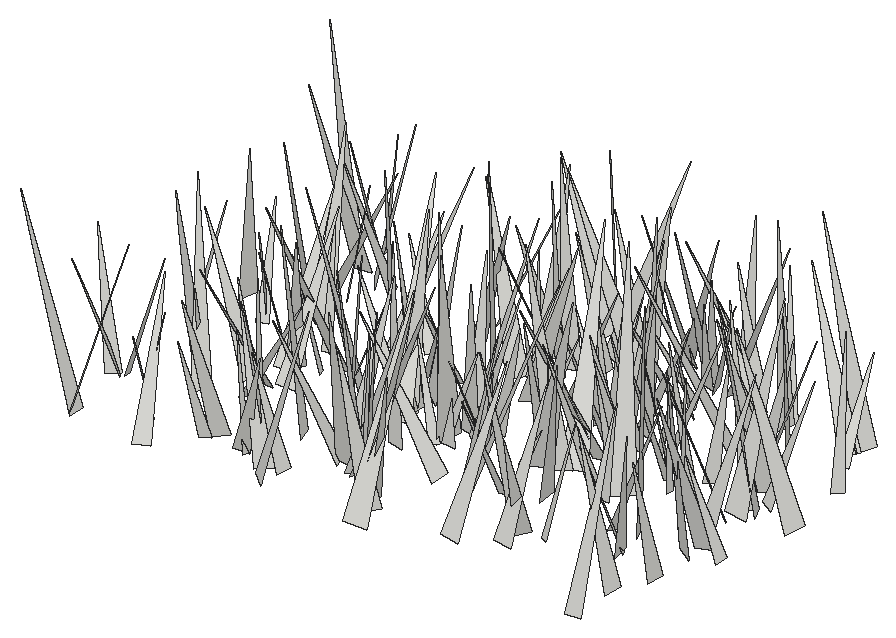
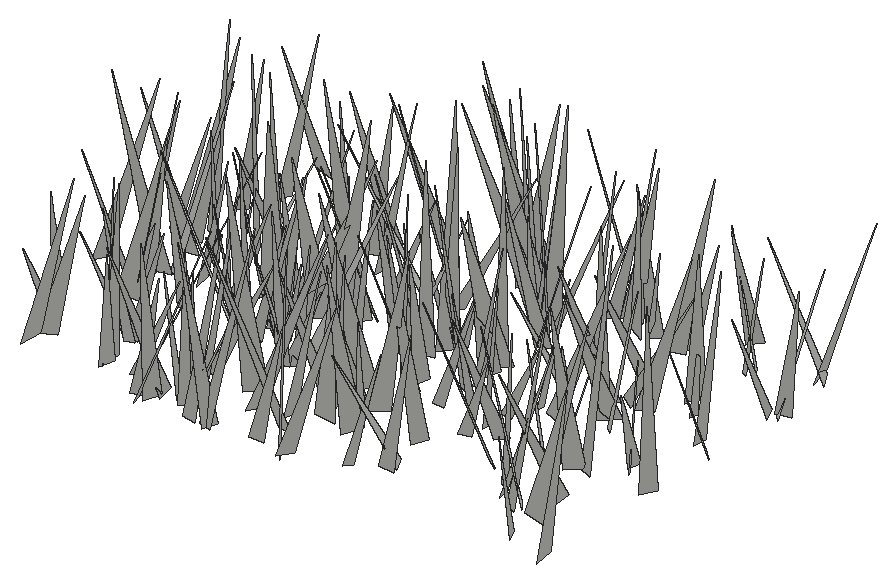
# SketchUp Ruby script. Lengths in inches.
U = 1.inch
M = Sketchup.active_model
def pt(a) = Geom::Point3d.new(a.map { |v| v * U })
def face(e, loops, mat)
  f = e.add_face(loops[0].map { |a| pt(a) })
  loops[1..].each { |l| e.add_face(l.map { |a| pt(a) }).erase! }
  f.material = f.back_material = mat if mat
  f
end
# faces: each face lists its corners as indices into pts; further lists are holes
def faces(e, pts, list, mat = nil) = list.each { |f| face(e, (f[0].is_a?(Array) ? f : [f]).map { |l| l.map { |i| pts[i] } }, mat) }
# xy, xz, yz: faces in a plane at the given z, y or x. An outline is a flat list of corners, or four numbers for a rectangle; further outlines are holes
def ring(l) = l.size == 4 ? [[l[0], l[1]], [l[2], l[1]], [l[2], l[3]], [l[0], l[3]]] : l.each_slice(2).to_a
def flat(e, list, mat, &to3) = list.each { |f| face(e, (f[0].is_a?(Array) ? f : [f]).map { |l| ring(l).map { |u, v| to3.(u, v) } }, mat) }
def xy(e, z, list, mat = nil) = flat(e, list, mat) { |x, y| [x, y, z] }
def xz(e, y, list, mat = nil) = flat(e, list, mat) { |x, z| [x, y, z] }
def yz(e, x, list, mat = nil) = flat(e, list, mat) { |y, z| [x, y, z] }
def lines(e, pts, list) = list.each { |a, b| e.add_line(pt(pts[a]), pt(pts[b])) }
# prism: a flat outline (further loops are holes) pulled along v
def prism(e, loops, v, mat = nil)
  f = face(e, loops, mat); d = Geom::Vector3d.new(v.map { |x| x * U })
  f.pushpull(f.normal.samedirection?(d) ? d.length : -d.length)
end
def box(e, o, s, mat = nil) = prism(e, [[o, [o[0] + s[0], o[1], o[2]], [o[0] + s[0], o[1] + s[1], o[2]], [o[0], o[1] + s[1], o[2]]]], [0, 0, s[2]], mat)
def at(x, y, z, deg = 0) = Geom::Transformation.translation(pt([x, y, z])) * Geom::Transformation.rotation(ORIGIN, Z_AXIS, deg.degrees)
def axes(o, x, y, z) = Geom::Transformation.new([*x, 0, *y, 0, *z, 0, *pt(o).to_a, 1])
def part(name) = M.definitions.add(name)
# library, detail: a bought-in or finely detailed component or shape, given as its bounding box
def library(name, o, s) = part(name).tap { |d| box(d.entities, o, s) }
def detail(e, o, s) = box(e.add_group.entities, o, s)
def put(e, d, t, mat = nil) = e.add_instance(d, t).tap { |i| i.material = mat if mat }
def group(e, t, mat = nil) = e.add_group.tap { |g| g.transformation = t; g.material = mat if mat }.entities
root = M.entities
c1 = part("fur_instance\#9")
p = [[0.8125,0,1.79],[0.67,-0.02,1.48],[0,-0.11,0],[0,0.11,0]]
faces(c1.entities,p,[[0,1,2,3]])
put(root,c1,axes([455.83,105.99,-21.66],[-7.51977,-1.08655,0.44758],[-1.14316,7.43533,-1.15625],[0.27218,1.20961,7.50937]))
put(root,c1,axes([478.6,107.64,-21.66],[3.4747,-4.84053,2.29693],[-4.84614,-4.00697,-1.11322],[-2.28507,1.13736,5.85363]))
put(root,c1,axes([470.41,106.39,-21.66],[4.17066,5.06918,1.33611],[5.23853,-4.09478,-0.81653],[-0.19883,-1.55319,6.51339]))
put(root,c1,axes([461.78,105.19,-21.66],[-3.2921,4.67046,0.35788],[4.62081,3.30978,-0.68745],[0.76768,0.10645,5.67261]))
put(root,c1,axes([478.07,108.55,-21.66],[6.05752,-0.57817,0.88939],[-0.39,-6.0087,-1.2499],[-0.9865,-1.17476,5.9553]))
put(root,c1,axes([459.88,108.68,-21.66],[-2.01295,-3.23513,0.63988],[-3.06607,2.112,1.03257],[1.21439,-0.03018,3.66768]))
put(root,c1,axes([467.22,108.6,-21.66],[2.01974,-4.62687,0.27657],[-4.52399,-1.90214,1.21619],[1.00891,0.73329,4.89981]))
put(root,c1,axes([459.48,107.97,-21.66],[4.05743,2.55482,1.17911],[2.80714,-3.81746,-1.3882],[-0.19333,-1.81108,4.58942]))
put(root,c1,axes([471.05,108.2,-21.66],[3.41803,-2.18502,2.15563],[-1.95303,-4.03718,-0.99543],[-2.36786,0.1758,3.93273]))
put(root,c1,axes([465.02,109.28,-21.66],[2.93992,-5.13493,1.13143],[-5.01799,-3.12719,-1.15379],[-1.5708,0.37938,5.8034]))
put(root,c1,axes([464.36,108.5,-21.66],[0.87067,-3.63818,0.96208],[-3.64876,-1.05785,-0.69825],[-0.92116,0.75142,3.67517]))
put(root,c1,axes([455.3125,106.12,-21.66],[5.06961,3.19969,0.78256],[3.08145,-5.11429,0.94868],[-1.16407,0.39664,5.91937]))
put(root,c1,axes([497.24,104.99,-21.66],[1.20703,6.81999,0.05967],[6.70849,-1.19813,1.23829],[-1.22962,0.158,6.81439]))
put(root,c1,axes([469.2,109.23,-21.66],[-5.69321,-2.11736,2.09192],[-1.78965,6.04293,1.24584],[2.37833,-0.52131,5.94506]))
put(root,c1,axes([478.99,105.47,-21.66],[-1.14842,8.02715,0.79991],[8.02073,1.22255,-0.75306],[0.86188,-0.68125,8.07384]))
put(root,c1,axes([478,107.31,-21.66],[7.83085,1.1219,1.78667],[1.00117,-8.02181,0.64907],[-1.85702,0.40616,7.88414]))
put(root,c1,axes([478.03,107.39,-21.66],[2.88835,4.68484,1.93004],[4.79823,-3.24275,0.69058],[-1.62782,-1.24585,5.46016]))
put(root,c1,axes([469.86,107.73,-21.66],[-2.9661,5.6248,1.68099],[5.86235,2.73802,1.18234],[-0.31135,-2.03143,6.24805]))
put(root,c1,axes([497.25,109.08,-21.66],[-5.83631,0.9789,1.84731],[1.28037,6.00401,0.86359],[1.65271,-1.19453,5.85448]))
put(root,c1,axes([476.66,109.51,-21.66],[6.37942,2.61315,2.43113],[3.05762,-6.56979,-0.96169],[-1.84118,-1.85616,6.82648]))
put(root,c1,axes([473.53,111.4,-21.66],[0.50064,-7.21064,0.91051],[-7.21991,-0.3887,0.89157],[0.83387,0.96363,7.17281]))
put(root,c1,axes([467.76,108.44,-21.66],[-4.02809,-0.22088,0.67447],[-0.39433,3.92835,-1.06856],[0.59008,1.11738,3.89005]))
put(root,c1,axes([488.08,111.35,-21.66],[3.42227,-3.49613,0.30492],[-3.40506,-3.41104,-0.89344],[-0.84941,-0.41195,4.81005]))
put(root,c1,axes([484.82,107.88,-21.66],[0.10942,6.44965,1.02032],[6.44115,0.06102,-1.07648],[1.07264,-1.02435,6.36012]))
put(root,c1,axes([468.54,108.96,-21.66],[2.01081,5.29668,2.07869],[5.40677,-2.46554,1.0522],[-1.77275,-1.51176,5.56697]))
put(root,c1,axes([454.66,111.86,-21.66],[-3.71629,-3.62879,0.54604],[-3.4741,3.72939,1.13989],[1.18191,-0.44788,5.0675]))
put(root,c1,axes([472.95,111.67,-21.66],[-5.60277,-1.40853,0.55452],[-1.25772,5.51462,1.29985],[0.84237,-1.13469,5.62898]))
put(root,c1,axes([474.89,110.81,-21.66],[5.41416,-4.66063,0.97473],[-4.76032,-5.26587,1.26282],[0.1044,1.59183,7.03135]))
put(root,c1,axes([487.88,109.47,-21.66],[-0.68675,5.73435,1.62653],[5.78722,1.03346,-1.2],[1.42703,-1.4315,5.64928]))
put(root,c1,axes([498.39,111.98,-21.66],[4.51587,-1.82573,1.61231],[-1.49442,-4.75873,-1.20297],[-1.92343,-0.58918,4.72009]))
put(root,c1,axes([484.13,109.28,-21.66],[4.06792,5.19434,1.22411],[5.14399,-4.22635,0.83955],[-1.42088,-0.42943,6.54403]))
put(root,c1,axes([454.54,111.4,-21.66],[-2.06507,4.56305,1.47225],[4.79287,1.92061,0.77009],[-0.13147,-1.65628,4.94903]))
put(root,c1,axes([474.97,110.89,-21.66],[7.79072,-0.23447,0.87822],[-0.35324,-7.76347,1.06082],[-0.83754,1.09323,7.72172]))
put(root,c1,axes([486.36,112.78,-21.66],[-6.02473,-0.71032,1.74625],[-0.51818,6.24626,0.75302],[1.81257,-0.57532,6.01954]))
put(root,c1,axes([494.53,113.22,-21.66],[5.27182,0.13194,1.25121],[0.40362,-5.28245,-1.14356],[-1.19165,-1.2055,5.14798]))
put(root,c1,axes([474.9,111.47,-21.66],[-4.32916,0.66549,1.27706],[0.40908,4.44763,-0.93094],[1.38073,0.76884,4.27993]))
put(root,c1,axes([474.12,112.22,-21.66],[-5.98871,-2.33617,1.80164],[-2.60473,6.10133,-0.74665],[1.38529,1.37273,6.38474]))
put(root,c1,axes([472.31,113.12,-21.66],[5.33637,4.77614,2.80857],[5.34994,-5.45601,-0.88678],[-1.44141,-2.56842,7.10647]))
put(root,c1,axes([469.09,112.7,-21.66],[-6.68963,-2.36331,2.10659],[-2.62997,6.88987,-0.62215],[1.76244,1.31094,7.06748]))
put(root,c1,axes([479.42,113.69,-21.66],[-6.11827,1.22354,0.04324],[1.20265,5.96505,1.37981],[-0.22923,-1.36132,6.08493]))
put(root,c1,axes([455.33,111.8,-21.66],[3.79033,1.52401,0.8214],[1.29616,-3.80865,1.0854],[-1.14773,0.73179,3.93842]))
put(root,c1,axes([489.63,111.56,-21.66],[2.15657,3.40289,0.33157],[3.29952,-2.17412,0.8525],[-0.89598,0.18416,3.93747]))
put(root,c1,axes([494.66,113.41,-21.66],[-3.19994,-2.12817,0.10035],[-2.08753,3.09569,-0.91527],[-0.42587,0.81635,3.73243]))
put(root,c1,axes([483.8,114.61,-21.66],[-1.02707,-3.52995,0.46815],[-3.49734,0.90838,-0.82343],[-0.66956,0.66999,3.58293]))
put(root,c1,axes([458.94,115,-21.66],[3.4639,-0.21189,1.20284],[0.06017,-3.58323,-0.80448],[-1.21988,-0.7784,3.37584]))
put(root,c1,axes([497.77,115.72,-21.66],[-3.27673,-6.38483,2.25273],[-6.55108,3.62196,0.73666],[1.71005,1.64109,7.13865]))
put(root,c1,axes([462.99,114.27,-21.66],[4.12414,-1.44643,0.07491],[-1.4095,-3.95608,1.21201],[0.33327,1.1677,4.19901]))
put(root,c1,axes([486.26,116.03,-21.66],[6.1777,-0.38175,1.16241],[-0.13775,-6.16226,-1.29169],[-1.21571,-1.24165,6.0532]))
put(root,c1,axes([498.44,117.05,-21.66],[1.25653,-6.81976,0.6894],[-6.81087,-1.32116,-0.65555],[-0.77223,0.55558,6.90349]))
put(root,c1,axes([460.31,113.14,-21.66],[-6.55915,2.85076,0.80174],[2.70921,6.56329,-1.17278],[1.19574,0.76707,7.05506]))
put(root,c1,axes([472.05,114.02,-21.66],[-0.35457,5.93898,1.63328],[6.05839,0.63143,-0.98081],[1.11129,-1.54746,5.86815]))
put(root,c1,axes([463.4,116.24,-21.66],[-2.21504,-4.22644,0.02495],[-4.06696,2.12371,-1.31133],[-1.15036,0.62998,4.58799]))
put(root,c1,axes([500.15,116.52,-21.66],[-3.89042,0.9571,1.21715],[1.27935,3.84105,1.06884],[0.87221,-1.36496,3.86121]))
put(root,c1,axes([474.51,115.24,-21.66],[1.78909,6.44129,2.50482],[6.73985,-2.19865,0.83993],[-1.52927,-2.15428,6.63216]))
put(root,c1,axes([461.87,116.39,-21.66],[-5.02266,3.34128,1.54054],[3.64584,4.87057,1.32283],[0.49523,-1.96924,5.88569]))
put(root,c1,axes([476.65,118.08,-21.66],[7.55718,-3.05255,1.8054],[-2.7949,-7.74218,-1.39129],[-2.18313,-0.65505,8.03077]))
put(root,c1,axes([481.8,113.76,-21.66],[5.80303,5.01805,0.27093],[4.96083,-5.78629,0.91567],[-0.80277,0.51711,7.61693]))
put(root,c1,axes([492.18,115.33,-21.66],[4.56042,0.58445,0.815],[0.35248,-4.48653,1.24501],[-0.93891,1.15443,4.42595]))
put(root,c1,axes([456.45,117.49,-21.66],[-5.67591,-0.59927,2.29984],[-0.30227,6.08824,0.84044],[2.35734,-0.66225,5.64524]))
put(root,c1,axes([493.87,116,-21.66],[-6.60957,-3.13791,3.29203],[-3.79035,7.01015,-0.92809],[2.51341,2.31982,7.25752]))
put(root,c1,axes([488.53,118.39,-21.66],[-5.81258,-1.56867,1.18702],[-1.32265,5.85738,1.26392],[1.45614,-0.94136,5.88637]))
put(root,c1,axes([470.77,117.24,-21.66],[-7.3033,-3.33888,1.09507],[-3.45877,7.27632,-0.88176],[0.61989,1.26191,7.98178]))
put(root,c1,axes([463.27,119.11,-21.66],[5.23311,-3.59302,0.50013],[-3.53385,-5.24745,-0.7222],[-0.81967,-0.31597,6.30664]))
put(root,c1,axes([483.375,118.81,-21.66],[5.39011,-5.98506,0.75501],[-6.02641,-5.29691,1.03406],[0.27067,1.25142,7.9878]))
put(root,c1,axes([479.37,118.42,-21.66],[3.73813,0.01426,0.67221],[0.17612,-3.68545,-0.90117],[-0.64889,-0.91811,3.62791]))
put(root,c1,axes([476.63,117.61,-21.66],[-0.2038,-3.57727,1.86557],[-3.68837,0.92217,1.36537],[1.63497,1.63446,3.31273]))
put(root,c1,axes([479.48,118.4,-21.66],[-3.75562,-3.58045,0.3486],[-3.58145,3.67402,-0.84892],[-0.33818,0.85312,5.11895]))
put(root,c1,axes([489.34,117.875,-21.66],[1.31397,-3.56018,1.31098],[-3.78942,-1.16427,0.63629],[0.18405,1.44556,3.7412]))
put(root,c1,axes([484.41,118.41,-21.66],[3.50873,2.55931,1.93983],[3.03472,-3.58228,-0.76287],[-1.05048,-1.80039,4.27543]))
put(root,c1,axes([469.1875,116.22,-21.66],[3.38601,2.0667,0.33408],[1.88033,-3.28152,1.24252],[-0.92044,0.89903,3.76728]))
put(root,c1,axes([476.36,116.92,-21.66],[-0.98772,3.5916,0.11089],[3.35733,0.88143,1.35606],[-1.28071,-0.45933,3.46934]))
put(root,c1,axes([476.99,117.36,-21.66],[1.25442,7.48082,2.76942],[7.81491,-1.71475,1.09211],[-1.59984,-2.51056,7.50623]))
put(root,c1,axes([477.25,119.49,-21.66],[0.11264,-6.37998,1.60761],[-6.5012,0.13924,1.0081],[1.01142,1.60553,6.30084]))
put(root,c1,axes([462.07,119.83,-21.66],[-3.11173,-3.4795,0.92655],[-3.33661,3.24675,0.98692],[1.3537,0.0043,4.56244]))
put(root,c1,axes([482.78,117.72,-21.66],[3.70587,4.25797,0.60198],[4.28884,-3.60158,-0.92773],[0.31394,-1.06043,5.56805]))
put(root,c1,axes([495.72,117.89,-21.66],[2.53366,4.26731,1.78001],[4.34271,-2.89305,0.75426],[-1.5872,-1.10369,4.90515]))
put(root,c1,axes([496.5,121.25,-21.66],[-4.09518,-5.32392,0.52178],[-5.17841,4.11019,1.29512],[1.34181,-0.38619,6.5907]))
put(root,c1,axes([465.73,120.85,-21.66],[-1.54524,-6.7658,0.51217],[-6.71547,1.44992,-1.10738],[-0.96994,0.74015,6.85109]))
put(root,c1,axes([464.27,116.77,-21.66],[-1.14169,6.19263,0.48775],[6.13199,1.20279,-0.91762],[0.99261,-0.30768,6.22978]))
put(root,c1,axes([478.04,118.76,-21.66],[3.54049,4.95211,1.34575],[5.12044,-3.30078,-1.32493],[0.33991,-1.85767,5.94164]))
put(root,c1,axes([467.2,120.37,-21.66],[-4.25466,-1.2014,1.34721],[-0.93808,4.41863,0.97784],[1.54219,-0.62673,4.31153]))
put(root,c1,axes([484.75,119.3,-21.66],[1.79805,-6.87497,3.712],[-7.43664,-2.674,-1.35027],[-2.39594,3.14033,6.97674]))
put(root,c1,axes([497.25,118.47,-21.66],[1.23681,5.98503,1.54047],[6.1022,-0.934,-1.27052],[0.97821,-1.7408,5.97797]))
put(root,c1,axes([478.81,120.27,-21.66],[3.21186,-3.52218,0.8528],[-3.62385,-3.13,0.72104],[-0.02677,1.11644,4.71189]))
put(root,c1,axes([464.93,119.6875,-21.66],[-3.69691,-1.68274,0.52652],[-1.75981,3.59718,-0.85985],[0.10916,1.00233,3.96981]))
put(root,c1,axes([485.88,122.02,-21.66],[-1.10699,-6.38687,0.31821],[-6.26084,1.01671,-1.37367],[-1.30201,0.54128,6.33487]))
put(root,c1,axes([455.16,118.375,-21.66],[3.04107,3.48011,0.59696],[3.3547,-3.09349,0.94446],[-1.10161,0.1866,4.52408]))
put(root,c1,axes([472.42,119,-21.66],[-5.70861,3.53079,2.01517],[3.32922,6.05385,-1.17592],[2.33318,0.00055,6.60847]))
put(root,c1,axes([481.35,121.64,-21.66],[4.6906,-0.13116,1.94102],[0.35682,-4.92253,-1.19491],[-1.91244,-1.24013,4.53774]))
put(root,c1,axes([487.46,121.46,-21.66],[3.16597,-2.82128,1.36449],[-2.73379,-3.43456,-0.75836],[-1.53229,0.2984,4.17228]))
put(root,c1,axes([487.93,122.07,-21.66],[2.45481,-4.16097,0.8917],[-4.06011,-2.59844,-0.9479],[-1.27449,0.26329,4.73722]))
put(root,c1,axes([472.73,119.92,-21.66],[-6.0397,-1.24718,1.08354],[-1.47294,5.92489,-1.39057],[0.74831,1.59618,6.00831]))
put(root,c1,axes([462.74,118.53,-21.66],[-1.71935,6.00909,0.23442],[5.94835,1.73522,-0.85232],[0.8839,0.01135,6.19184]))
put(root,c1,axes([472.59,117.78,-21.66],[-4.41357,6.91206,0.00056],[6.86097,4.38103,-0.99489],[0.83882,0.53496,8.14041]))
put(root,c1,axes([472.5,121.53,-21.66],[-2.78435,-5.66723,3.39056],[-5.97834,3.72634,1.319],[2.80584,2.3158,6.17497]))
put(root,c1,axes([486.87,122.82,-21.66],[-3.71631,2.59474,2.95715],[3.6126,3.86147,1.15179],[1.55775,-2.76492,4.38373]))
put(root,c1,axes([489.99,119.22,-21.66],[-7.18499,4.19207,1.05141],[4.04317,7.24035,-1.23823],[1.52698,0.55406,8.22584]))
put(root,c1,axes([494.46,120.93,-21.66],[-5.51822,-0.21879,0.79161],[-0.32668,5.51842,-0.75206],[0.75352,0.79022,5.4711]))
put(root,c1,axes([501.37,122.53,-21.66],[-7.04891,1.70289,1.4017],[1.92518,7.04086,1.12767],[1.07622,-1.44158,7.16347]))
put(root,c1,axes([492.04,121.45,-21.66],[-3.53666,-0.44387,1.07965],[-0.6619,3.59984,-0.68824],[0.96154,0.84544,3.49732]))
put(root,c1,axes([490.95,122.54,-21.66],[-2.05485,-3.90462,0.97999],[-3.96047,1.76344,-1.27819],[-0.72186,1.43981,4.22312]))
put(root,c1,axes([486.05,122.87,-21.66],[-2.14589,-4.13922,0.79032],[-4.13009,1.88974,-1.31675],[-0.83673,1.28775,4.4726]))
put(root,c1,axes([457.51,123.41,-21.66],[3.15596,1.30372,1.61225],[1.82364,-3.14251,-1.02861],[-0.98659,-1.6383,3.25603]))
put(root,c1,axes([470.65,123.1,-21.66],[3.7872,-0.0255,0.26622],[0.02172,-3.73751,-0.66706],[-0.26655,-0.66693,3.72808]))
put(root,c1,axes([483.1,124.13,-21.66],[-4.92734,-5.46841,0.2776],[-5.45988,4.87887,-0.80338],[-0.41255,0.74316,7.31688]))
put(root,c1,axes([498.1,122.74,-21.66],[-6.28358,-3.49392,1.76213],[-3.72095,6.36668,-0.64478],[1.21124,1.43309,7.16066]))
put(root,c1,axes([472.57,124.1,-21.66],[0.53786,-3.60504,0.14249],[-3.55289,-0.5543,-0.6129],[-0.62738,0.04841,3.59304]))
put(root,c1,axes([485.4375,119.86,-21.66],[-4.43994,6.98412,0.3729],[6.94517,4.45476,-0.74146],[0.82561,0.08476,8.24265]))
put(root,c1,axes([468.29,122.52,-21.66],[-1.80359,3.13263,0.44398],[3.00697,1.53819,1.36218],[-0.98418,-1.04117,3.34825]))
put(root,c1,axes([497.26,121.59,-21.66],[0.16612,7.76506,1.97129],[7.95416,0.07536,-0.96713],[0.95574,-1.97685,7.70638]))
put(root,c1,axes([463.5,122.04,-21.66],[0.00503,4.167,0.7042],[4.17874,-0.11,0.62111],[-0.63075,-0.69557,4.12045]))
put(root,c1,axes([468.43,124.45,-21.66],[4.23217,0.79223,1.75299],[1.35483,-4.23497,-1.35698],[-1.36567,-1.74623,4.08626]))
put(root,c1,axes([459.77,125.11,-21.66],[-3.5221,-6.63629,1.77015],[-6.5539,3.84233,1.36448],[2.0543,0.8804,7.38808]))
put(root,c1,axes([489.56,124.32,-21.66],[-3.13954,-2.86345,1.03549],[-2.74612,3.30524,0.81394],[1.31545,0.06589,4.17056]))
put(root,c1,axes([475.31,122.42,-21.66],[-4.49774,2.41965,1.22715],[2.26445,4.65664,-0.88215],[1.49428,0.22634,5.03052]))
put(root,c1,axes([454.97,124.63,-21.66],[5.79339,-2.08626,1.56673],[-1.97661,-6.00002,-0.68061],[-1.70297,-0.13319,6.11985]))
put(root,c1,axes([496.99,125.39,-21.66],[1.49882,-6.76146,1.59023],[-6.75855,-1.79498,-1.262],[-1.60255,1.24632,6.80963]))
put(root,c1,axes([487.15,124.48,-21.66],[-0.77658,-4.10323,1.17838],[-4.23531,0.59015,-0.73621],[-0.53592,1.28194,4.11067]))
put(root,c1,axes([457.85,122.44,-21.66],[-3.33951,2.40161,0.05247],[2.31618,3.24301,-1.02031],[0.63702,0.79874,3.98485]))
put(root,c1,axes([497.44,122.75,-21.66],[-6.80477,1.06742,0.77743],[0.9228,6.76292,-1.20833],[0.94457,1.0827,6.78117]))
put(root,c1,axes([493.25,124.06,-21.66],[3.51253,-2.51047,1.78394],[-2.89575,-3.6135,0.61652],[-1.0486,1.56939,4.2732]))
put(root,c1,axes([482.89,125.7,-21.66],[3.48904,-1.79502,0.75996],[-1.60226,-3.52839,-0.97792],[-1.11014,-0.54905,3.7999]))
put(root,c1,axes([488.62,124.55,-21.66],[2.69077,3.3772,1.27263],[3.60609,-2.57991,-0.77814],[-0.14558,-1.48455,4.24737]))
put(root,c1,axes([498.06,123.8125,-21.66],[2.30047,4.4169,0.81433],[4.47004,-2.16262,-0.89782],[0.43686,-1.13065,4.89848]))
put(root,c1,axes([487.16,122.99,-21.66],[4.31579,6.0344,1.65644],[5.97789,-4.5707,1.07586],[-1.85004,-0.69181,7.34048]))
put(root,c1,axes([475.23,122.89,-21.66],[4.30738,5.01035,0.65824],[4.94004,-4.35705,0.83813],[-1.06435,0.05398,6.55397]))
put(root,c1,axes([477.54,125.19,-21.66],[5.60342,-3.67276,1.04707],[-3.81273,-5.48708,1.15708],[-0.22057,1.54484,6.59914]))
put(root,c1,axes([489.59,124.07,-21.66],[4.90909,4.36789,0.50992],[4.39704,-4.86378,-0.66882],[0.06695,-0.83837,6.53684]))
put(root,c1,axes([475.34,124.32,-21.66],[-6.98093,-2.98191,2.95578],[-3.56155,7.24267,-1.10492],[2.22346,2.23913,7.51028]))
put(root,c1,axes([485.04,124.03,-21.66],[-4.58169,-0.00231,0.33908],[-0.10273,4.38765,-1.35823],[0.32316,1.36211,4.37574]))
put(root,c1,axes([483.6,126.2,-21.66],[0.23103,-4.99246,1.62863],[-5.17408,0.0623,0.92493],[0.89778,1.64376,4.91147]))
put(root,c1,axes([483.45,125.6875,-21.66],[-2.38468,3.13652,0.12042],[3.02513,2.25628,1.13874],[-0.83714,-0.7813,3.77197]))
put(root,c1,axes([491.6,128.34,-21.66],[-6.74137,-3.47517,0.05647],[-3.44773,6.70195,0.85032],[0.43951,-0.73012,7.53656]))
put(root,c1,axes([484.39,124.89,-21.66],[3.67967,2.76321,1.03507],[2.46473,-3.78797,1.35021],[-1.62229,0.51247,4.39911]))
put(root,c1,axes([466.65,125.04,-21.66],[-1.32926,4.80497,0.97182],[4.66035,1.55098,-1.29408],[1.52094,-0.553,4.81456]))
put(root,c1,axes([460.62,125.17,-21.66],[-3.43213,5.64571,1.59286],[5.69776,3.64732,-0.65059],[1.39526,-1.00684,6.57497]))
put(root,c1,axes([468.8125,126.11,-21.66],[-2.26305,3.25436,0.20739],[3.19812,2.16563,0.91504],[-0.63708,-0.68879,3.8568]))
put(root,c1,axes([486.45,126.0625,-21.66],[3.17531,6.56755,2.54139],[6.79761,-3.58673,0.77578],[-1.83954,-1.91744,7.25351]))
put(root,c1,axes([470.55,128.56,-21.66],[6.6655,-1.52718,0.22941],[-1.49066,-6.62814,-0.81212],[-0.40351,-0.74118,6.78982]))
put(root,c1,axes([485.29,127.11,-21.66],[4.11337,-1.35782,0.42666],[-1.42017,-4.00175,0.95638],[-0.09392,1.04301,4.22479]))
put(root,c1,axes([475.1,127,-21.66],[-5.2406,4.407,1.34408],[4.57378,5.22157,0.71269],[0.55566,-1.41624,6.81011]))
put(root,c1,axes([479.43,127.07,-21.66],[4.44559,-0.41699,0.42413],[-0.48383,-4.39553,0.74982],[-0.34594,0.78895,4.4017]))
put(root,c1,axes([459.94,128.62,-21.66],[4.41125,2.39111,1.26664],[2.67652,-4.21168,-1.37073],[-0.39751,-1.82353,4.82677]))
put(root,c1,axes([475.95,127.3,-21.66],[1.17442,4.10835,0.87727],[4.16659,-1.02282,-0.78793],[0.5364,-1.0501,4.19964]))
put(root,c1,axes([493.22,129.625,-21.66],[1.75124,-3.26229,0.83742],[-3.12175,-1.92651,-0.97669],[-1.26432,0.23809,3.57148]))
put(root,c1,axes([486.37,129.98,-21.66],[-0.29394,-4.28793,0.2812],[-4.0742,0.18848,-1.38464],[-1.36614,0.36048,4.06885]))
put(root,c1,axes([486.57,130.38,-21.66],[-3.34858,-4.98605,1.16696],[-4.83329,3.53804,1.24784],[1.69169,0.23891,5.87509]))
put(root,c1,axes([462.59,129.77,-21.66],[-2.53313,-4.37285,1.78451],[-4.47538,2.86942,0.67851],[1.50904,1.16947,5.00781]))
put(root,c1,axes([475.53,128.41,-21.66],[-3.90689,0.46662,1.17538],[0.26281,4.03296,-0.72751],[1.23701,0.61693,3.86682]))
put(root,c1,axes([465.07,127.97,-21.66],[3.93505,4.96293,0.50565],[4.97977,-3.8695,-0.7745],[0.29702,-0.87596,6.28613]))
put(root,c1,axes([462.05,130.61,-21.66],[-5.06877,-1.96642,0.89661],[-1.81084,5.11214,0.97466],[1.17965,-0.60192,5.34876]))
put(root,c1,axes([477.48,128.41,-21.66],[-6.31895,-1.30533,1.91515],[-1.71826,6.37081,-1.32708],[1.5554,1.73484,6.31441]))
put(root,c1,axes([500.5,128.02,-21.66],[-4.9436,1.78617,0.77223],[1.56135,4.89918,-1.33648],[1.16143,1.01666,5.08364]))
put(root,c1,axes([460.6,131.74,-21.66],[-3.28751,-5.48957,1.02333],[-5.33666,3.43821,1.29963],[1.64396,0.18343,6.2653]))
put(root,c1,axes([494.35,130.57,-21.66],[-4.3896,-2.50757,2.34029],[-2.3133,4.97071,0.98703],[2.5325,0.19407,4.95805]))
put(root,c1,axes([458.72,128.68,-21.66],[4.92318,-0.35306,0.35659],[-0.43613,-4.74982,1.31852],[-0.24819,1.34315,4.75646]))
put(root,c1,axes([493.17,129.97,-21.66],[0.04539,-4.24616,1.86431],[-4.44886,0.48634,1.21602],[1.30888,1.80033,4.06857]))
put(root,c1,axes([482.85,129.96,-21.66],[-2.73382,6.12597,3.74599],[6.6709,3.64992,-1.10045],[2.6569,-2.86083,6.61742]))
put(root,c1,axes([486.19,131.41,-21.66],[-3.41179,-1.77285,0.16017],[-1.67154,3.30984,1.02951],[0.61205,-0.84317,3.70451]))
put(root,c1,axes([479.12,131.07,-21.66],[-5.12264,0.34016,1.65759],[0.60899,5.30124,0.79415],[1.57874,-0.94118,5.07212]))
put(root,c1,axes([494.16,129.09,-21.66],[3.89284,1.77366,0.49192],[1.64576,-3.86945,0.92782],[-0.82421,0.65077,4.17603]))
put(root,c1,axes([458.6,131.83,-21.66],[-0.74223,-7.02206,1.66779],[-7.14663,0.48084,-1.156],[-1.00829,1.76103,6.96591]))
put(root,c1,axes([477.17,129.97,-21.66],[-0.74799,6.94474,2.29097],[7.27165,0.46217,0.97314],[-0.77532,-2.36525,6.91678]))
put(root,c1,axes([481.41,131.76,-21.66],[-7.37091,1.53228,0.84327],[1.65266,7.29739,1.18581],[0.57246,-1.33774,7.43452]))
put(root,c1,axes([460.25,130.98,-21.66],[4.87544,3.99495,1.42226],[4.19795,-4.85335,-0.75795],[-0.59966,-1.4959,6.2574]))
put(root,c1,axes([474.77,130.15,-21.66],[-5.03968,3.97301,2.20808],[3.85689,5.48236,-1.06156],[2.40517,-0.46656,6.329]))
put(root,c1,axes([485.34,133.625,-21.66],[-0.07367,-4.26522,0.50041],[-4.16979,0.19077,1.01214],[1.02732,0.46845,4.14405]))
put(root,c1,axes([469.96,132.71,-21.66],[-0.83956,4.61048,2.28414],[5.1209,0.52371,0.82514],[-0.50027,-2.37653,4.61309]))
put(root,c1,axes([498.55,130.86,-21.66],[-1.96871,3.37657,0.07437],[3.27614,1.93014,-0.90775],[0.82077,0.39482,3.80171]))
put(root,c1,axes([490.25,132.89,-21.66],[-3.73947,1.85603,0.44676],[1.90802,3.6015,1.00834],[-0.06253,-1.10111,4.05114]))
put(root,c1,axes([485.99,133.73,-21.66],[4.14097,0.37336,0.37849],[0.46882,-3.96604,-1.21698],[-0.25072,-1.24957,3.97567]))
put(root,c1,axes([472.2,133.77,-21.66],[-3.76395,0.54517,1.33918],[0.93594,3.7652,1.09781],[1.1021,-1.33566,3.64133]))
put(root,c1,axes([485.17,134.28,-21.66],[0.2797,-5.08952,0.70223],[-5.01624,-0.11848,1.13926],[1.11073,0.74654,4.96825]))
put(root,c1,axes([497.95,132.41,-21.66],[-4.76226,4.46867,0.77555],[4.53262,4.64929,1.04363],[-0.16086,-1.29026,6.44663]))
put(root,c1,axes([492.59,132.55,-21.66],[-6.8831,0.44539,2.18741],[0.27023,7.20464,-0.61666],[2.21588,0.50489,6.86987]))
put(root,c1,axes([482.55,135.5625,-21.66],[-2.90954,-6.16313,0.64564],[-6.10361,2.97343,0.8781],[1.07095,0.20243,6.75859]))
put(root,c1,axes([469.79,131.65,-21.66],[4.40688,2.08061,0.00975],[2.02682,-4.29803,1.08102],[-0.47012,0.97349,4.75194]))
put(root,c1,axes([488.1,135.54,-21.66],[-5.70608,-2.81682,0.48614],[-2.67601,5.6456,1.30244],[1.0049,-0.96065,6.22877]))
put(root,c1,axes([483.9,135.46,-21.66],[-1.823,-5.96341,0.88128],[-5.94354,1.93183,0.77754],[1.00658,0.60664,6.18716]))
put(root,c1,axes([482.34,135.3,-21.66],[6.03259,-1.06555,0.38284],[-1.02373,-6.01977,-0.62323],[-0.48366,-0.54868,6.09418]))
put(root,c1,axes([492.49,133.11,-21.66],[-4.5808,2.50643,0.71678],[2.42315,4.62824,-0.69815],[0.96142,0.27723,5.1748]))
put(root,c1,axes([478.18,132.74,-21.66],[3.15625,6.97995,0.87784],[7.00121,-3.02246,-1.14023],[0.68808,-1.26383,7.57506]))
put(root,c1,axes([498.39,133.55,-21.66],[-7.87651,1.28049,0.44694],[1.23259,7.85729,-0.78901],[0.56579,0.70864,7.94081]))
put(root,c1,axes([476.51,135.4,-21.66],[-4.90081,-4.60842,2.76686],[-4.75517,5.4628,0.67611],[2.50627,1.35324,6.69315]))
put(root,c1,axes([488.52,134.91,-21.66],[-2.55012,3.64542,1.48438],[3.93085,2.44958,0.73729],[0.20222,-1.64502,4.38733]))
put(root,c1,axes([487.19,133.75,-21.66],[5.64038,0.84844,0.8162],[0.68974,-5.61874,1.07421],[-0.95409,0.95384,5.60177]))
put(root,c1,axes([478.86,134.86,-21.66],[-2.03282,4.17049,1.29504],[4.34211,1.77825,1.08919],[-0.46493,-1.62705,4.50988]))
put(root,c1,axes([476.25,135.15,-21.66],[-6.01632,2.22797,0.81671],[2.32649,5.97644,0.83455],[0.46722,-1.07014,6.36109]))
put(root,c1,axes([458.35,134.34,-21.66],[-3.5127,-1.06556,1.8883],[-1.54789,3.74984,-0.76344],[1.51826,1.35772,3.59049]))
put(root,c1,axes([487.5,134.73,-21.66],[4.97353,-2.18793,2.98402],[-2.79783,-5.49524,0.634],[-2.42149,1.85546,5.39639]))
put(root,c1,axes([454.93,135.375,-21.66],[-7.05246,-0.20222,1.59365],[-0.38202,7.18084,-0.77939],[1.56034,0.84409,7.01218]))
